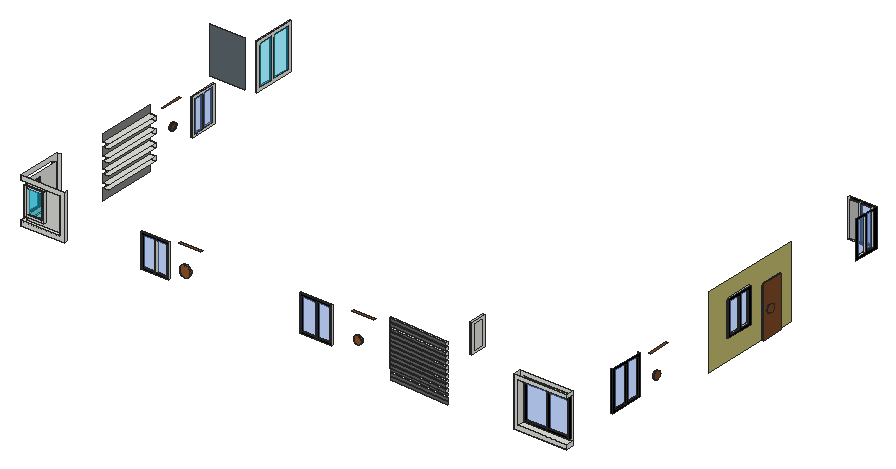
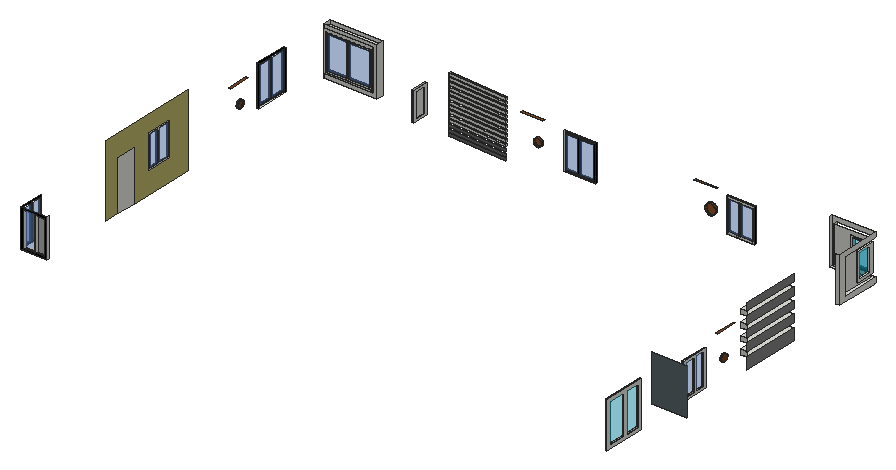
# SketchUp Ruby script. Lengths in inches.
U = 1.inch
M = Sketchup.active_model
def pt(a) = Geom::Point3d.new(a.map { |v| v * U })
def face(e, loops, mat)
  f = e.add_face(loops[0].map { |a| pt(a) })
  loops[1..].each { |l| e.add_face(l.map { |a| pt(a) }).erase! }
  f.material = f.back_material = mat if mat
  f
end
# faces: each face lists its corners as indices into pts; further lists are holes
def faces(e, pts, list, mat = nil) = list.each { |f| face(e, (f[0].is_a?(Array) ? f : [f]).map { |l| l.map { |i| pts[i] } }, mat) }
# xy, xz, yz: faces in a plane at the given z, y or x. An outline is a flat list of corners, or four numbers for a rectangle; further outlines are holes
def ring(l) = l.size == 4 ? [[l[0], l[1]], [l[2], l[1]], [l[2], l[3]], [l[0], l[3]]] : l.each_slice(2).to_a
def flat(e, list, mat, &to3) = list.each { |f| face(e, (f[0].is_a?(Array) ? f : [f]).map { |l| ring(l).map { |u, v| to3.(u, v) } }, mat) }
def xy(e, z, list, mat = nil) = flat(e, list, mat) { |x, y| [x, y, z] }
def xz(e, y, list, mat = nil) = flat(e, list, mat) { |x, z| [x, y, z] }
def yz(e, x, list, mat = nil) = flat(e, list, mat) { |y, z| [x, y, z] }
def lines(e, pts, list) = list.each { |a, b| e.add_line(pt(pts[a]), pt(pts[b])) }
# prism: a flat outline (further loops are holes) pulled along v
def prism(e, loops, v, mat = nil)
  f = face(e, loops, mat); d = Geom::Vector3d.new(v.map { |x| x * U })
  f.pushpull(f.normal.samedirection?(d) ? d.length : -d.length)
end
def box(e, o, s, mat = nil) = prism(e, [[o, [o[0] + s[0], o[1], o[2]], [o[0] + s[0], o[1] + s[1], o[2]], [o[0], o[1] + s[1], o[2]]]], [0, 0, s[2]], mat)
def at(x, y, z, deg = 0) = Geom::Transformation.translation(pt([x, y, z])) * Geom::Transformation.rotation(ORIGIN, Z_AXIS, deg.degrees)
def axes(o, x, y, z) = Geom::Transformation.new([*x, 0, *y, 0, *z, 0, *pt(o).to_a, 1])
def part(name) = M.definitions.add(name)
# library, detail: a bought-in or finely detailed component or shape, given as its bounding box
def library(name, o, s) = part(name).tap { |d| box(d.entities, o, s) }
def detail(e, o, s) = box(e.add_group.entities, o, s)
def put(e, d, t, mat = nil) = e.add_instance(d, t).tap { |i| i.material = mat if mat }
def group(e, t, mat = nil) = e.add_group.tap { |g| g.transformation = t; g.material = mat if mat }.entities
root = M.entities
M.materials.add("[0057_DarkKhaki]").color = [189, 183, 107]
M.materials.add("[0133_Gray]").color = [128, 128, 128]
M.materials.add("[0134_DimGray]").color = [105, 105, 105]
M.materials.add("[0137_Black]").color = [0, 0, 0]
M.materials.add("[Formica Speckled Grey]").color = [94, 105, 111]
M.materials.add("[Mirror 01]").color = [185, 185, 185]
M.materials.add("[Translucent Glass Blue]").color = [100, 149, 237]
M.materials["[Translucent Glass Blue]"].alpha = 0.5
M.materials.add("[Translucent Glass Tinted]").color = [8, 201, 241]
M.materials["[Translucent Glass Tinted]"].alpha = 0.48
M.materials.add("[Wood Cherry Original]").color = [152, 86, 42]
M.materials.add("[Wood Veneer 01]").color = [120, 70, 37]
xy(root,133.12,[[972.47,541.6875,975.47,577.6875]])
xy(root,146.59,[[80.8125,480.26,83.8125,524.95]])
xy(root,147.13,[[884.72,140.58,972.47,152.58]])
xy(root,148.55,[[74.8125,620.4,77.8125,690.23]])
xy(root,149.59,[[80.8125,483.26,83.8125,499.85],[80.8125,502.6,83.8125,521.95]])
xy(root,152.94,[[519.3,155.58,572.17,158.58]])
xy(root,153.62,[[83.8125,295.24,92.8125,392.06]])
xy(root,153.81,[[74.8125,625.66,77.8125,650.5],[74.8125,655.3125,77.8125,684.97]])
xy(root,154.54,[[891.83,140.58,972.47,152.58]])
xy(root,154.86,[[766.19,148.96,667.84,154.96,668.06,158.52,766.41,152.52]])
xy(root,155.5,[[257.26,155.58,303.45,158.58]])
xy(root,155.94,[[522.3,155.58,545.74,158.58],[549.49,155.58,569.17,158.58]],"[0137_Black]")
xy(root,156.3,[[893.13,149.58,968.57,152.58]])
xy(root,158.5,[[260.26,155.58,280.35,158.58],[282.85,155.58,300.45,158.58]],"[0137_Black]")
xy(root,158.875,[[68.8125,149.58,74.8125,219.58]])
xy(root,159.06,[[766.19,148.96,766.41,152.52,668.06,158.52,667.84,154.96]])
xy(root,159.09,[[68.8125,143.58,141.375,149.58]])
xy(root,159.3,[[896.13,149.58,930.85,152.58],[933.66,149.58,965.57,152.58]],"[0137_Black]")
xy(root,161.05,[[972.47,230.95,975.47,286.51]])
xy(root,161.06,[[83.8125,295.24,92.8125,392.06]])
xy(root,161.73,[[766.19,148.96,667.84,154.96,668.06,158.52,766.41,152.52]])
xy(root,164.05,[[972.47,233.95,975.47,258.73],[972.47,260.87,975.47,283.51]],"[0137_Black]")
xy(root,165.93,[[766.19,148.96,766.41,152.52,668.06,158.52,667.84,154.96]])
xy(root,166.6,[[931.72,770.48,972.47,773.48],[972.47,770.48,975.47,773.48]])
xy(root,167.09,[[68.8125,143.58,74.8125,209.08],[74.8125,143.58,133.51,149.58]])
xy(root,167.95,[[972.47,469.23,975.47,514.23]])
xy(root,168.61,[[766.19,148.96,667.84,154.96,668.06,158.52,766.41,152.52]])
xy(root,169.6,[[934.72,770.48,949.25,773.48],[952.09,770.48,969.47,773.48]],"[0137_Black]")
xy(root,170.15,[[972.47,735.23,975.47,751.36],[972.47,754.32,975.47,767.48]])
xy(root,170.95,[[972.47,472.23,975.47,491.73],[972.47,494.52,975.47,511.23]],"[0137_Black]")
xy(root,172.81,[[766.19,148.96,766.41,152.52,668.06,158.52,667.84,154.96]])
xy(root,172.89,[[71.8125,149.58,74.8125,178.02]])
xy(root,172.97,[[71.8125,146.58,105.375,149.58]])
xy(root,173.56,[[83.8125,295.24,92.8125,392.06]])
xy(root,175.48,[[766.19,148.96,667.84,154.96,668.06,158.52,766.41,152.52]])
xy(root,175.89,[[71.8125,152.58,74.8125,175.02]])
xy(root,175.97,[[77.8125,146.58,102.375,149.58]])
xy(root,179.68,[[766.19,148.96,766.41,152.52,668.06,158.52,667.84,154.96]])
xy(root,181,[[83.8125,295.24,92.8125,392.06]])
xy(root,182.36,[[766.19,148.96,667.84,154.96,668.06,158.52,766.41,152.52]])
xy(root,186.56,[[766.19,148.96,766.41,152.52,668.06,158.52,667.84,154.96]])
xy(root,187.6,[[763.41,201.89,766.41,227.45]])
xy(root,189.23,[[766.19,148.96,667.84,154.96,668.06,158.52,766.41,152.52]])
xy(root,190.6,[[763.41,204.89,766.41,224.45]])
xy(root,193.43,[[766.19,148.96,766.41,152.52,668.06,158.52,667.84,154.96]])
xy(root,193.5,[[83.8125,295.24,92.8125,392.06]])
xy(root,196.11,[[766.19,148.96,667.84,154.96,668.06,158.52,766.41,152.52]])
xy(root,200.31,[[766.19,148.96,766.41,152.52,668.06,158.52,667.84,154.96]])
xy(root,200.94,[[83.8125,295.24,92.8125,392.06]])
xy(root,202.78,[[80.8125,483.26,83.8125,499.85],[80.8125,502.6,83.8125,521.95]])
xy(root,202.98,[[766.19,148.96,667.84,154.96,668.06,158.52,766.41,152.52]])
xy(root,205.78,[[80.8125,480.26,83.8125,524.95]])
xy(root,207.18,[[766.19,148.96,766.41,152.52,668.06,158.52,667.84,154.96]])
xy(root,207.62,[[260.26,155.58,280.35,158.58],[282.85,155.58,300.45,158.58]],"[0137_Black]")
xy(root,209.25,[[522.3,155.58,545.74,158.58],[549.49,155.58,569.17,158.58]],"[0137_Black]")
xy(root,209.86,[[766.19,148.96,667.84,154.96,668.06,158.52,766.41,152.52]])
xy(root,210.62,[[257.26,155.58,303.45,158.58]],"[0137_Black]")
xy(root,212.25,[[519.3,155.58,572.17,158.58]],"[0137_Black]")
xy(root,213.43,[[83.8125,295.24,92.8125,392.06]])
xy(root,214.06,[[766.19,148.96,766.41,152.52,668.06,158.52,667.84,154.96]])
xy(root,214.42,[[896.13,149.58,930.85,152.58],[933.66,149.58,965.57,152.58]],"[0137_Black]")
xy(root,215.91,[[77.8125,146.58,102.375,149.58],[71.8125,152.58,74.8125,175.02]])
xy(root,216.18,[[321.0625,155.58,357.0625,158.58],[605.91,155.58,641.91,158.58]],"[Wood Cherry Original]")
xy(root,216.18,[[972.47,308.49,975.47,344.49],[80.8125,419.71,83.8125,455.71],[972.47,541.6875,975.47,577.6875]],"[Wood Veneer 01]")
xy(root,216.73,[[766.19,148.96,667.84,154.96,668.06,158.52,766.41,152.52]])
xy(root,217.42,[[893.13,149.58,968.57,152.58]],"[0137_Black]")
xy(root,218.87,[[74.8125,625.66,77.8125,650.5],[74.8125,655.3125,77.8125,684.97]])
xy(root,218.91,[[71.8125,146.58,105.375,146.58,105.375,149.58,74.8125,149.58,74.8125,178.02,71.8125,178.02]])
xy(root,220.88,[[83.8125,295.24,92.8125,392.06]])
xy(root,220.93,[[766.19,148.96,766.41,152.52,668.06,158.52,667.84,154.96]])
xy(root,221.82,[[891.83,140.58,972.47,152.58]])
xy(root,222.63,[[972.47,472.23,975.47,491.73],[972.47,494.52,975.47,511.23]])
xy(root,223.61,[[766.19,148.96,667.84,154.96,668.06,158.52,766.41,152.52]])
xy(root,224.05,[[972.47,233.95,975.47,258.73],[972.47,260.87,975.47,283.51]])
xy(root,224.13,[[74.8125,620.4,77.8125,690.23]])
xz(root,140.58,[[884.72,147.13,972.47,147.13,972.47,154.54,891.83,154.54,891.83,221.82,972.47,221.82,972.47,227.94,884.72,227.94]])
xz(root,143.58,[[68.8125,159.09,141.375,159.09,141.375,233.3125,68.8125,233.3125,68.8125,225.8125,133.51,225.8125,133.51,167.09,68.8125,167.09]])
xz(root,146.58,[[[71.8125,172.97,105.375,218.91],[77.8125,175.97,102.375,215.91]]])
xz(root,149.58,[[74.8125,167.09,133.51,167.09,133.51,225.8125,68.8125,225.8125,68.8125,225.75,74.8125,225.75,74.8125,218.91,105.375,218.91,105.375,172.97,71.8125,172.97,71.8125,172.89,74.8125,172.89]])
xz(root,149.58,[[[893.13,156.3,968.57,217.42],[896.13,159.3,930.85,214.42],[933.66,159.3,965.57,214.42]]],"[0137_Black]")
xz(root,149.58,[[77.8125,175.97,102.375,215.91]],"[Translucent Glass Tinted]")
xz(root,152.58,[[884.72,147.13,884.72,227.94,972.47,227.94,972.47,221.82,891.83,221.82,891.83,154.54,972.47,154.54,972.47,147.13],[[891.83,154.54,972.47,221.82],[893.13,156.3,968.57,217.42]],[[893.13,156.3,968.57,217.42],[896.13,159.3,930.85,214.42],[933.66,159.3,965.57,214.42]],[71.8125,175.89,74.8125,215.91]])
xz(root,152.58,[[896.13,159.3,930.85,214.42],[933.66,159.3,965.57,214.42]],"[Translucent Glass Blue]")
xz(root,152.58,[[332.67,170.77,335,171.08,337.17,171.97,339.03,173.4,340.46,175.27,341.36,177.4375,341.67,179.77,341.36,182.1,340.46,184.27,339.03,186.13,337.17,187.5625,335,188.46,332.67,188.77,330.34,188.46,328.17,187.5625,326.31,186.13,324.875,184.27,323.98,182.1,323.67,179.77,323.98,177.4375,324.875,175.27,326.31,173.4,328.17,171.97,330.34,171.08],[617.1875,171.51,618.9,171.73,620.5,172.39,621.87,173.45,622.92,174.82,623.59,176.42,623.8125,178.13,623.59,179.84,622.92,181.44,621.87,182.81,620.5,183.87,618.9,184.53,617.1875,184.76,615.47,184.53,613.875,183.87,612.5,182.81,611.45,181.44,610.79,179.84,610.5625,178.13,610.79,176.42,611.45,174.82,612.5,173.45,613.875,172.39,615.47,171.73]],"[Wood Cherry Original]")
xz(root,155.58,[[[519.3,152.94,572.17,212.25],[522.3,155.94,545.74,209.25],[549.49,155.94,569.17,209.25]],[[257.26,155.5,303.45,210.62],[260.26,158.5,280.35,207.62],[282.85,158.5,300.45,207.62]]],"[0137_Black]")
xz(root,158.58,[[[257.26,155.5,303.45,210.62],[260.26,158.5,280.35,207.62],[282.85,158.5,300.45,207.62]]])
xz(root,158.58,[[522.3,155.94,545.74,209.25],[549.49,155.94,569.17,209.25],[260.26,158.5,280.35,207.62],[282.85,158.5,300.45,207.62]],"[Translucent Glass Blue]")
xz(root,175.02,[[71.8125,175.89,74.8125,215.91]])
xz(root,178.02,[[71.8125,172.89,74.8125,218.91]])
xz(root,201.89,[[763.41,187.6,766.41,235.22]])
xz(root,204.89,[[763.41,190.6,766.41,232.22]])
xz(root,209.08,[[68.8125,167.09,74.8125,225.75]])
xz(root,219.58,[[68.8125,158.875,74.8125,233.3125]])
xz(root,224.45,[[763.41,190.6,766.41,232.22]])
xz(root,227.45,[[763.41,187.6,766.41,235.22]])
xz(root,230.95,[[972.47,161.05,975.47,227.05]],"[0137_Black]")
xz(root,233.95,[[972.47,164.05,975.47,224.05]],"[0137_Black]")
xz(root,258.73,[[972.47,164.05,975.47,224.05]],"[0137_Black]")
xz(root,260.87,[[972.47,164.05,975.47,224.05]],"[0137_Black]")
xz(root,283.51,[[972.47,164.05,975.47,224.05]],"[0137_Black]")
xz(root,286.51,[[972.47,161.05,975.47,227.05]],"[0137_Black]")
xz(root,392.06,[[83.8125,153.62,92.8125,161.06],[83.8125,173.56,92.8125,181],[83.8125,193.5,92.8125,200.94],[83.8125,213.43,92.8125,220.88]])
xz(root,469.23,[[972.47,167.95,975.47,225.63]],"[0137_Black]")
xz(root,472.23,[[972.47,170.95,975.47,222.63]],"[0137_Black]")
xz(root,480.26,[[80.8125,146.59,83.8125,205.78]])
xz(root,483.26,[[80.8125,149.59,83.8125,202.78]])
xz(root,491.73,[[972.47,170.95,975.47,222.63]],"[0137_Black]")
xz(root,494.52,[[972.47,170.95,975.47,222.63]],"[0137_Black]")
xz(root,499.85,[[80.8125,149.59,83.8125,202.78]])
xz(root,502.6,[[80.8125,149.59,83.8125,202.78]])
xz(root,511.23,[[972.47,170.95,975.47,222.63]],"[0137_Black]")
xz(root,514.23,[[972.47,167.95,975.47,225.63]],"[0137_Black]")
xz(root,521.95,[[80.8125,149.59,83.8125,202.78]])
xz(root,524.95,[[80.8125,146.59,83.8125,205.78]])
xz(root,541.6875,[[972.47,133.12,975.47,216.18]],"[Wood Veneer 01]")
xz(root,577.6875,[[972.47,133.12,975.47,216.18]],"[Wood Veneer 01]")
xz(root,587.65,[[26.03,169.22,83.8125,246.18]],"[Formica Speckled Grey]")
xz(root,620.4,[[74.8125,148.55,77.8125,224.13]])
xz(root,625.66,[[74.8125,153.81,77.8125,218.87]])
xz(root,650.5,[[74.8125,153.81,77.8125,218.87]])
xz(root,655.3125,[[74.8125,153.81,77.8125,218.87]])
xz(root,684.97,[[74.8125,153.81,77.8125,218.87]])
xz(root,690.23,[[74.8125,148.55,77.8125,224.13]])
xz(root,735.23,[[972.47,170.15,975.47,226.04]],"[0137_Black]")
xz(root,751.36,[[972.47,170.15,975.47,226.04]])
xz(root,754.32,[[972.47,170.15,975.47,226.04]],"[0137_Black]")
xz(root,767.48,[[972.47,170.15,975.47,226.04]])
xz(root,770.48,[[934.72,169.6,949.25,226.04]],"[Mirror 01]")
xz(root,770.48,[[952.09,169.6,969.47,226.04]],"[Translucent Glass Blue]")
xz(root,773.48,[[[931.72,166.6,975.47,229.04],[952.09,169.6,969.47,226.04],[934.72,169.6,949.25,226.04]]],"[0137_Black]")
yz(root,68.8125,[[149.58,158.875,149.58,159.09,143.58,159.09,143.58,167.09,209.08,167.09,209.08,225.75,149.58,225.75,149.58,225.8125,143.58,225.8125,143.58,233.3125,219.58,233.3125,219.58,158.875]])
yz(root,71.8125,[[[149.58,172.89,149.58,172.97,146.58,172.97,146.58,218.91,178.02,218.91,178.02,172.89],[152.58,175.89,175.02,215.91]]])
yz(root,74.8125,[[[620.4,148.55,690.23,224.13],[655.3125,153.81,684.97,218.87],[625.66,153.81,650.5,218.87]],[149.58,167.09,149.58,172.89,178.02,172.89,178.02,218.91,149.58,218.91,149.58,225.75,209.08,225.75,209.08,167.09]])
yz(root,74.8125,[[152.58,175.89,175.02,215.91]],"[Translucent Glass Tinted]")
yz(root,77.8125,[[[620.4,148.55,690.23,224.13],[655.3125,153.81,684.97,218.87],[625.66,153.81,650.5,218.87]],[146.58,175.97,149.58,215.91]])
yz(root,77.8125,[[625.66,153.81,650.5,218.87],[655.3125,153.81,684.97,218.87]],"[Translucent Glass Tinted]")
yz(root,77.8125,[[444.54,170.94,443.07,171.13,441.7,171.7,440.52,172.61,439.61,173.78,439.05,175.16,438.85,176.63,439.05,178.1,439.61,179.47,440.52,180.65,441.7,181.55,443.07,182.12,444.54,182.32,446.01,182.12,447.38,181.55,448.5625,180.65,449.47,179.47,450.03,178.1,450.23,176.63,450.03,175.16,449.47,173.78,448.5625,172.61,447.38,171.7,446.01,171.13]],"[Wood Veneer 01]")
yz(root,80.8125,[[[480.26,146.59,524.95,205.78],[502.6,149.59,521.95,202.78],[483.26,149.59,499.85,202.78]]])
yz(root,83.8125,[[[480.26,146.59,524.95,205.78],[502.6,149.59,521.95,202.78],[483.26,149.59,499.85,202.78]]])
yz(root,83.8125,[[295.24,133.68,392.06,153.62],[295.24,161.06,392.06,173.56],[295.24,181,392.06,193.5],[295.24,200.94,392.06,213.43],[295.24,220.88,392.06,233.37]],"[0133_Gray]")
yz(root,83.8125,[[483.26,149.59,499.85,202.78],[502.6,149.59,521.95,202.78]],"[Translucent Glass Blue]")
yz(root,102.375,[[146.58,175.97,149.58,215.91]])
yz(root,105.375,[[146.58,172.97,149.58,218.91]])
yz(root,133.51,[[143.58,167.09,149.58,225.8125]])
yz(root,141.375,[[143.58,159.09,149.58,233.3125]])
yz(root,257.26,[[155.58,155.5,158.58,210.62]],"[0137_Black]")
yz(root,260.26,[[155.58,158.5,158.58,207.62]],"[0137_Black]")
yz(root,280.35,[[155.58,158.5,158.58,207.62]],"[0137_Black]")
yz(root,282.85,[[155.58,158.5,158.58,207.62]])
yz(root,300.45,[[155.58,158.5,158.58,207.62]],"[0137_Black]")
yz(root,303.45,[[155.58,155.5,158.58,210.62]])
yz(root,519.3,[[155.58,152.94,158.58,212.25]],"[0137_Black]")
yz(root,522.3,[[155.58,155.94,158.58,209.25]],"[0137_Black]")
yz(root,545.74,[[155.58,155.94,158.58,209.25]],"[0137_Black]")
yz(root,549.49,[[155.58,155.94,158.58,209.25]],"[0137_Black]")
yz(root,569.17,[[155.58,155.94,158.58,209.25]],"[0137_Black]")
yz(root,572.17,[[155.58,152.94,158.58,212.25]])
yz(root,763.41,[[[201.89,187.6,227.45,235.22],[204.89,190.6,224.45,232.22]]])
yz(root,766.41,[[[201.89,187.6,227.45,235.22],[204.89,190.6,224.45,232.22]],[204.89,190.6,224.45,232.22]])
yz(root,884.72,[[140.58,147.13,152.58,227.94]])
yz(root,891.83,[[140.58,154.54,152.58,221.82]])
yz(root,893.13,[[149.58,156.3,152.58,217.42]],"[0137_Black]")
yz(root,896.13,[[149.58,159.3,152.58,214.42]],"[0137_Black]")
yz(root,930.85,[[149.58,159.3,152.58,214.42]],"[0137_Black]")
yz(root,931.72,[[770.48,166.6,773.48,229.04]])
yz(root,933.66,[[149.58,159.3,152.58,214.42]],"[0137_Black]")
yz(root,934.72,[[770.48,169.6,773.48,226.04]],"[Translucent Glass Blue]")
yz(root,949.25,[[770.48,169.6,773.48,226.04]])
yz(root,952.09,[[770.48,169.6,773.48,226.04]],"[0137_Black]")
yz(root,965.57,[[149.58,159.3,152.58,214.42]],"[0137_Black]")
yz(root,968.57,[[149.58,156.3,152.58,217.42]],"[0137_Black]")
yz(root,969.47,[[770.48,169.6,773.48,226.04]])
yz(root,972.47,[[541.6875,133.12,577.6875,216.18],[140.58,147.13,152.58,154.54],[[469.23,167.95,514.23,225.63],[472.23,170.95,491.73,222.63],[494.52,170.95,511.23,222.63]],[140.58,221.82,152.58,227.94]])
yz(root,972.47,[[[431.23,133.12,541.6875,133.12,541.6875,216.18,577.6875,216.18,577.6875,133.12,600.85,133.12,600.85,252.18,431.23,252.18],[469.23,167.95,514.23,225.63]]],"[0057_DarkKhaki]")
yz(root,972.47,[[233.95,164.05,258.73,224.05],[260.87,164.05,283.51,224.05],[735.23,170.15,751.36,226.04],[754.32,170.15,767.48,226.04],[472.23,170.95,491.73,222.63],
  [494.52,170.95,511.23,222.63]],"[Translucent Glass Blue]")
yz(root,975.47,[[[230.95,161.05,286.51,227.05],[233.95,164.05,258.73,224.05],[260.87,164.05,283.51,224.05]],[[732.23,166.6,773.48,229.04],[735.23,170.15,751.36,226.04],[754.32,170.15,767.48,226.04]],[[469.23,167.95,514.23,225.63],[472.23,170.95,491.73,222.63],[494.52,170.95,511.23,222.63]]],"[0137_Black]")
yz(root,975.47,[[[541.6875,133.12,577.6875,216.18],[553.13,169.65,551.48,169.87,549.95,170.5,548.625,171.52,547.61,172.84,546.97,174.375,546.76,176.03,546.97,177.68,547.61,179.21,548.625,180.53,549.95,181.55,551.48,182.18,553.13,182.4,554.78,182.18,556.32,181.55,557.64,180.53,558.65,179.21,559.29,177.68,559.51,176.03,559.29,174.375,558.65,172.84,557.64,171.52,556.32,170.5,554.78,169.87]]],"[Wood Veneer 01]")
yz(root,978.47,[[553.13,169.65,554.78,169.87,556.32,170.5,557.64,171.52,558.65,172.84,559.29,174.375,559.51,176.03,559.29,177.68,558.65,179.21,557.64,180.53,556.32,181.55,554.78,182.18,553.13,182.4,551.48,182.18,549.95,181.55,548.625,180.53,547.61,179.21,546.97,177.68,546.76,176.03,546.97,174.375,547.61,172.84,548.625,171.52,549.95,170.5,551.48,169.87],[318.88,174.15,320.47,174.36,321.95,174.98,323.22,175.95,324.1875,177.22,324.8,178.69,325.01,180.28,324.8,181.86,324.1875,183.34,323.22,184.61,321.95,185.58,320.47,186.2,318.88,186.4,317.3,186.2,315.82,185.58,314.55,184.61,313.58,183.34,312.97,181.86,312.76,180.28,312.97,178.69,313.58,177.22,314.55,175.95,315.82,174.98,317.3,174.36]],"[Wood Veneer 01]")
p = [[766.41,152.52,139.18],[668.06,158.52,139.18],[668.06,158.52,134.98],[766.41,152.52,134.98],[766.41,152.52,145.18],[668.06,158.52,145.18],
  [668.06,158.52,140.98],[766.41,152.52,140.98],[766.41,152.52,152.18],[668.06,158.52,152.18],[668.06,158.52,147.98],[766.41,152.52,147.98],
  [766.19,148.96,159.06],[667.84,154.96,159.06],[667.84,154.96,154.86],[766.19,148.96,154.86],[766.41,152.52,154.86],[766.41,152.52,159.06],
  [668.06,158.52,159.06],[668.06,158.52,154.86],[766.19,148.96,165.93],[667.84,154.96,165.93],[667.84,154.96,161.73],[766.19,148.96,161.73],
  [766.41,152.52,161.73],[766.41,152.52,165.93],[668.06,158.52,165.93],[668.06,158.52,161.73],[766.19,148.96,172.81],[667.84,154.96,172.81],
  [667.84,154.96,168.61],[766.19,148.96,168.61],[766.41,152.52,168.61],[766.41,152.52,172.81],[668.06,158.52,172.81],[668.06,158.52,168.61],
  [975.47,551.48,169.87],[975.47,553.13,169.65],[978.47,553.13,169.65],[978.47,551.48,169.87],[975.47,554.78,169.87],[978.47,554.78,169.87],
  [975.47,549.95,170.5],[978.47,549.95,170.5],[975.47,556.32,170.5],[978.47,556.32,170.5],[975.47,548.625,171.52],[978.47,548.625,171.52],
  [975.47,557.64,171.52],[978.47,557.64,171.52],[330.34,155.58,171.08],[332.67,155.58,170.77],[332.67,152.58,170.77],[330.34,152.58,171.08],
  [335,155.58,171.08],[335,152.58,171.08],[80.8125,444.54,170.94],[80.8125,443.07,171.13],[77.8125,443.07,171.13],[77.8125,444.54,170.94],
  [80.8125,446.01,171.13],[77.8125,446.01,171.13],[328.17,155.58,171.97],[328.17,152.58,171.97],[337.17,155.58,171.97],[337.17,152.58,171.97],
  [80.8125,441.7,171.7],[77.8125,441.7,171.7],[80.8125,447.38,171.7],[77.8125,447.38,171.7],[615.47,155.58,171.73],[617.1875,155.58,171.51],
  [617.1875,152.58,171.51],[615.47,152.58,171.73],[618.9,155.58,171.73],[618.9,152.58,171.73],[975.47,547.61,172.84],[978.47,547.61,172.84],
  [975.47,558.65,172.84],[978.47,558.65,172.84],[613.875,155.58,172.39],[613.875,152.58,172.39],[620.5,155.58,172.39],[620.5,152.58,172.39],
  [80.8125,440.52,172.61],[77.8125,440.52,172.61],[80.8125,448.5625,172.61],[77.8125,448.5625,172.61],[326.31,155.58,173.4],[326.31,152.58,173.4],
  [339.03,155.58,173.4],[339.03,152.58,173.4],[612.5,155.58,173.45],[612.5,152.58,173.45],[621.87,155.58,173.45],[621.87,152.58,173.45],
  [80.8125,439.61,173.78],[77.8125,439.61,173.78],[80.8125,449.47,173.78],[77.8125,449.47,173.78],[975.47,546.97,174.375],[978.47,546.97,174.375],
  [975.47,559.29,174.375],[978.47,559.29,174.375],[324.875,155.58,175.27],[324.875,152.58,175.27],[340.46,155.58,175.27],[340.46,152.58,175.27],
  [611.45,155.58,174.82],[611.45,152.58,174.82],[622.92,155.58,174.82],[622.92,152.58,174.82],[80.8125,439.05,175.16],[77.8125,439.05,175.16],
  [80.8125,450.03,175.16],[77.8125,450.03,175.16],[975.47,317.3,174.36],[975.47,318.88,174.15],[978.47,318.88,174.15],[978.47,317.3,174.36],
  [975.47,320.47,174.36],[978.47,320.47,174.36],[975.47,315.82,174.98],[978.47,315.82,174.98],[975.47,321.95,174.98],[978.47,321.95,174.98],
  [975.47,546.76,176.03],[978.47,546.76,176.03],[975.47,559.51,176.03],[978.47,559.51,176.03],[610.79,155.58,176.42],[610.79,152.58,176.42],
  [623.59,155.58,176.42],[623.59,152.58,176.42],[975.47,314.55,175.95],[978.47,314.55,175.95],[975.47,323.22,175.95],[978.47,323.22,175.95],
  [80.8125,438.85,176.63],[77.8125,438.85,176.63],[80.8125,450.23,176.63],[77.8125,450.23,176.63],[323.98,155.58,177.4375],[323.98,152.58,177.4375],
  [341.36,155.58,177.4375],[341.36,152.58,177.4375],[766.19,148.96,179.68],[667.84,154.96,179.68],[667.84,154.96,175.48],[766.19,148.96,175.48],
  [766.41,152.52,175.48],[766.41,152.52,179.68],[668.06,158.52,179.68],[668.06,158.52,175.48],[975.47,313.58,177.22],[978.47,313.58,177.22],
  [975.47,324.1875,177.22],[978.47,324.1875,177.22],[975.47,546.97,177.68],[978.47,546.97,177.68],[975.47,559.29,177.68],[978.47,559.29,177.68],
  [610.5625,155.58,178.13],[610.5625,152.58,178.13],[623.8125,155.58,178.13],[623.8125,152.58,178.13],[80.8125,439.05,178.1],[77.8125,439.05,178.1],
  [80.8125,450.03,178.1],[77.8125,450.03,178.1],[975.47,312.97,178.69],[978.47,312.97,178.69],[975.47,324.8,178.69],[978.47,324.8,178.69],
  [323.67,155.58,179.77],[323.67,152.58,179.77],[341.67,155.58,179.77],[341.67,152.58,179.77],[975.47,547.61,179.21],[978.47,547.61,179.21],
  [975.47,558.65,179.21],[978.47,558.65,179.21],[610.79,155.58,179.84],[610.79,152.58,179.84],[623.59,155.58,179.84],[623.59,152.58,179.84],
  [80.8125,439.61,179.47],[77.8125,439.61,179.47],[80.8125,449.47,179.47],[77.8125,449.47,179.47],[975.47,312.76,180.28],[978.47,312.76,180.28],
  [975.47,325.01,180.28],[978.47,325.01,180.28],[975.47,548.625,180.53],[978.47,548.625,180.53],[975.47,557.64,180.53],[978.47,557.64,180.53],
  [80.8125,440.52,180.65],[77.8125,440.52,180.65],[80.8125,448.5625,180.65],[77.8125,448.5625,180.65],[323.98,155.58,182.1],[323.98,152.58,182.1],
  [341.36,155.58,182.1],[341.36,152.58,182.1],[611.45,155.58,181.44],[611.45,152.58,181.44],[622.92,155.58,181.44],[622.92,152.58,181.44],
  [975.47,312.97,181.86],[978.47,312.97,181.86],[975.47,324.8,181.86],[978.47,324.8,181.86],[975.47,549.95,181.55],[978.47,549.95,181.55],
  [975.47,556.32,181.55],[978.47,556.32,181.55],[80.8125,441.7,181.55],[77.8125,441.7,181.55],[80.8125,447.38,181.55],[77.8125,447.38,181.55],
  [612.5,155.58,182.81],[612.5,152.58,182.81],[621.87,155.58,182.81],[621.87,152.58,182.81],[975.47,551.48,182.18],[978.47,551.48,182.18],
  [975.47,554.78,182.18],[978.47,554.78,182.18],[80.8125,443.07,182.12],[77.8125,443.07,182.12],[80.8125,446.01,182.12],[77.8125,446.01,182.12],
  [975.47,313.58,183.34],[978.47,313.58,183.34],[975.47,324.1875,183.34],[978.47,324.1875,183.34],[324.875,155.58,184.27],[324.875,152.58,184.27],
  [340.46,155.58,184.27],[340.46,152.58,184.27],[80.8125,444.54,182.32],[77.8125,444.54,182.32],[975.47,553.13,182.4],[978.47,553.13,182.4],
  [766.19,148.96,186.56],[667.84,154.96,186.56],[667.84,154.96,182.36],[766.19,148.96,182.36],[766.41,152.52,182.36],[766.41,152.52,186.56],
  [668.06,158.52,186.56],[668.06,158.52,182.36],[613.875,155.58,183.87],[613.875,152.58,183.87],[620.5,155.58,183.87],[620.5,152.58,183.87],
  [975.47,314.55,184.61],[978.47,314.55,184.61],[975.47,323.22,184.61],[978.47,323.22,184.61],[615.47,155.58,184.53],[615.47,152.58,184.53],
  [618.9,155.58,184.53],[618.9,152.58,184.53],[326.31,155.58,186.13],[326.31,152.58,186.13],[339.03,155.58,186.13],[339.03,152.58,186.13],
  [617.1875,155.58,184.76],[617.1875,152.58,184.76],[975.47,315.82,185.58],[978.47,315.82,185.58],[975.47,321.95,185.58],[978.47,321.95,185.58],
  [975.47,317.3,186.2],[978.47,317.3,186.2],[975.47,320.47,186.2],[978.47,320.47,186.2],[328.17,155.58,187.5625],[328.17,152.58,187.5625],
  [337.17,155.58,187.5625],[337.17,152.58,187.5625],[975.47,318.88,186.4],[978.47,318.88,186.4],[330.34,155.58,188.46],[330.34,152.58,188.46],
  [335,155.58,188.46],[335,152.58,188.46],[332.67,155.58,188.77],[332.67,152.58,188.77],[766.19,148.96,193.43],[667.84,154.96,193.43],
  [667.84,154.96,189.23],[766.19,148.96,189.23],[766.41,152.52,189.23],[766.41,152.52,193.43],[668.06,158.52,193.43],[668.06,158.52,189.23],
  [766.19,148.96,200.31],[667.84,154.96,200.31],[667.84,154.96,196.11],[766.19,148.96,196.11],[766.41,152.52,196.11],[766.41,152.52,200.31],
  [668.06,158.52,200.31],[668.06,158.52,196.11],[766.19,148.96,207.18],[667.84,154.96,207.18],[667.84,154.96,202.98],[766.19,148.96,202.98],
  [766.41,152.52,202.98],[766.41,152.52,207.18],[668.06,158.52,207.18],[668.06,158.52,202.98],[766.19,148.96,214.06],[667.84,154.96,214.06],
  [667.84,154.96,209.86],[766.19,148.96,209.86],[766.41,152.52,209.86],[766.41,152.52,214.06],[668.06,158.52,214.06],[668.06,158.52,209.86],
  [766.19,148.96,220.93],[667.84,154.96,220.93],[667.84,154.96,216.73],[766.19,148.96,216.73],[766.41,152.52,216.73],[766.41,152.52,220.93],
  [668.06,158.52,220.93],[668.06,158.52,216.73],[766.19,148.96,227.81],[667.84,154.96,227.81],[667.84,154.96,223.61],[766.19,148.96,223.61],
  [766.41,152.52,223.61],[766.41,152.52,227.81],[668.06,158.52,227.81],[668.06,158.52,223.61],[-50.49,-92.45,186.67],[-50.49,-92.45,189.67]]
faces(root,p,[[0,1,2,3],[4,5,6,7],[8,9,10,11],[12,13,14,15],[20,21,22,23],[28,29,30,31],[146,147,148,149],[246,247,248,249],
  [292,293,294,295],[300,301,302,303],[308,309,310,311],[316,317,318,319],[324,325,326,327],[332,333,334,335]],"[0134_DimGray]")
faces(root,p,[[16,17,12,15],[18,17,16,19],[18,19,14,13],[24,25,20,23],[26,25,24,27],[26,27,22,21],[32,33,28,31],[34,33,32,35],
  [34,35,30,29],[150,151,146,149],[152,151,150,153],[152,153,148,147],[250,251,246,249],[252,251,250,253],[252,253,248,247],[296,297,292,295],
  [298,297,296,299],[298,299,294,293],[304,305,300,303],[306,305,304,307],[306,307,302,301],[312,313,308,311],[314,313,312,315],[314,315,310,309],
  [320,321,316,319],[322,321,320,323],[322,323,318,317],[328,329,324,327],[330,329,328,331],[330,331,326,325],[336,337,332,335],[338,337,336,339],
  [338,339,334,333]])
faces(root,p,[[36,37,38,39],[37,40,41,38],[42,36,39,43],[40,44,45,41],[46,42,43,47],[44,48,49,45],[56,57,58,59],[60,56,59,61],
  [57,66,67,58],[68,60,61,69],[76,46,47,77],[48,78,79,49],[66,84,85,67],[86,68,69,87],[84,96,97,85],[98,86,87,99],
  [100,76,77,101],[78,102,103,79],[96,112,113,97],[114,98,99,115],[116,117,118,119],[117,120,121,118],[122,116,119,123],[120,124,125,121],
  [126,100,101,127],[102,128,129,103],[134,122,123,135],[124,136,137,125],[112,138,139,113],[140,114,115,141],[154,134,135,155],[136,156,157,137],
  [158,126,127,159],[128,160,161,129],[138,166,167,139],[168,140,141,169],[170,154,155,171],[156,172,173,157],[178,158,159,179],[160,180,181,161],
  [166,186,187,167],[188,168,169,189],[190,170,171,191],[172,192,193,173],[194,178,179,195],[180,196,197,181],[186,198,199,187],[200,188,189,201],
  [210,190,191,211],[192,212,213,193],[214,194,195,215],[196,216,217,197],[198,218,219,199],[220,200,201,221],[226,214,215,227],[216,228,229,217],
  [218,230,231,219],[232,220,221,233],[234,210,211,235],[212,236,237,213],[230,242,243,231],[242,232,233,243],[244,226,227,245],[228,244,245,229],
  [258,234,235,259],[236,260,261,237],[272,258,259,273],[260,274,275,261],[276,272,273,277],[274,278,279,275],[284,276,277,285],[278,284,285,279]],"[Wood Veneer 01]")
faces(root,p,[[50,51,52,53],[51,54,55,52],[62,50,53,63],[54,64,65,55],[70,71,72,73],[71,74,75,72],[80,70,73,81],[74,82,83,75],
  [88,62,63,89],[64,90,91,65],[92,80,81,93],[82,94,95,83],[104,88,89,105],[90,106,107,91],[108,92,93,109],[94,110,111,95],
  [130,108,109,131],[110,132,133,111],[142,104,105,143],[106,144,145,107],[162,130,131,163],[132,164,165,133],[174,142,143,175],[144,176,177,145],
  [182,162,163,183],[164,184,185,165],[202,174,175,203],[176,204,205,177],[206,182,183,207],[184,208,209,185],[222,206,207,223],[208,224,225,209],
  [238,202,203,239],[204,240,241,205],[254,222,223,255],[224,256,257,225],[262,254,255,263],[256,264,265,257],[266,238,239,267],[240,268,269,241],
  [270,262,263,271],[264,270,271,265],[280,266,267,281],[268,282,283,269],[286,280,281,287],[282,288,289,283],[290,286,287,291],[288,290,291,289]],"[Wood Cherry Original]")
lines(root,p,[[340,341]])
